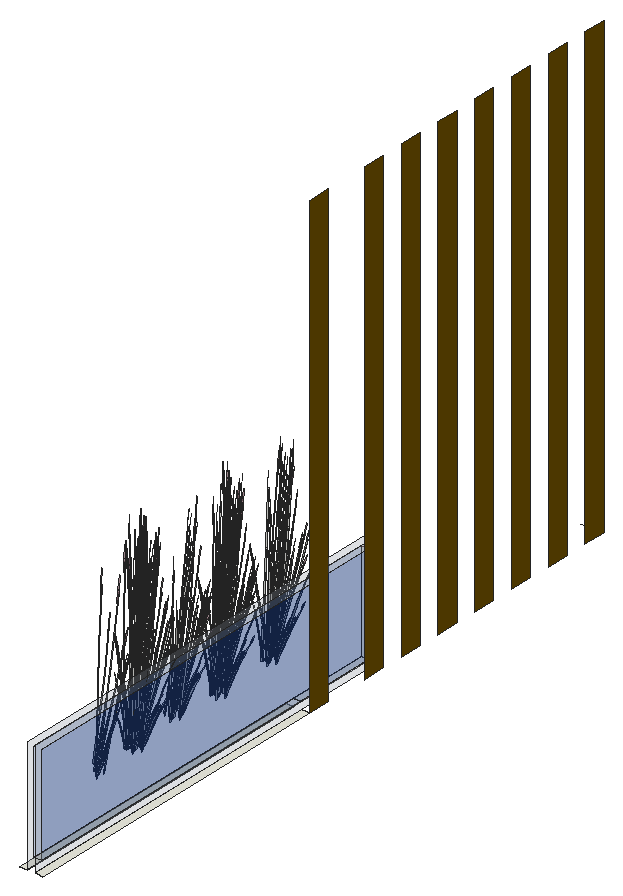
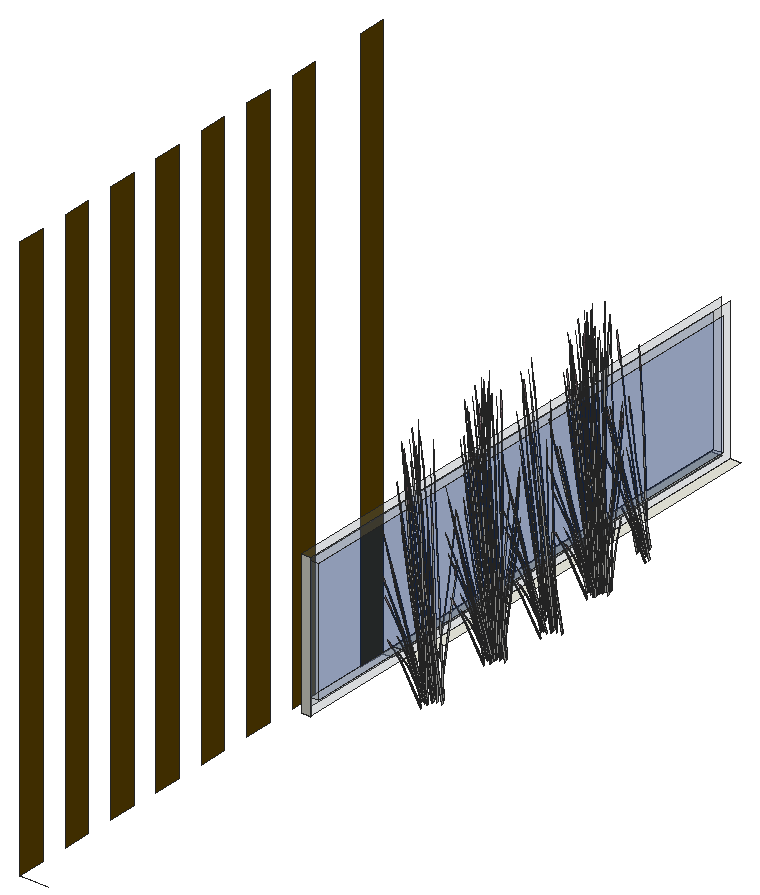
# SketchUp Ruby script. Lengths in inches.
U = 1.inch
M = Sketchup.active_model
def pt(a) = Geom::Point3d.new(a.map { |v| v * U })
def face(e, loops, mat)
  f = e.add_face(loops[0].map { |a| pt(a) })
  loops[1..].each { |l| e.add_face(l.map { |a| pt(a) }).erase! }
  f.material = f.back_material = mat if mat
  f
end
# faces: each face lists its corners as indices into pts; further lists are holes
def faces(e, pts, list, mat = nil) = list.each { |f| face(e, (f[0].is_a?(Array) ? f : [f]).map { |l| l.map { |i| pts[i] } }, mat) }
# xy, xz, yz: faces in a plane at the given z, y or x. An outline is a flat list of corners, or four numbers for a rectangle; further outlines are holes
def ring(l) = l.size == 4 ? [[l[0], l[1]], [l[2], l[1]], [l[2], l[3]], [l[0], l[3]]] : l.each_slice(2).to_a
def flat(e, list, mat, &to3) = list.each { |f| face(e, (f[0].is_a?(Array) ? f : [f]).map { |l| ring(l).map { |u, v| to3.(u, v) } }, mat) }
def xy(e, z, list, mat = nil) = flat(e, list, mat) { |x, y| [x, y, z] }
def xz(e, y, list, mat = nil) = flat(e, list, mat) { |x, z| [x, y, z] }
def yz(e, x, list, mat = nil) = flat(e, list, mat) { |y, z| [x, y, z] }
def lines(e, pts, list) = list.each { |a, b| e.add_line(pt(pts[a]), pt(pts[b])) }
# prism: a flat outline (further loops are holes) pulled along v
def prism(e, loops, v, mat = nil)
  f = face(e, loops, mat); d = Geom::Vector3d.new(v.map { |x| x * U })
  f.pushpull(f.normal.samedirection?(d) ? d.length : -d.length)
end
def box(e, o, s, mat = nil) = prism(e, [[o, [o[0] + s[0], o[1], o[2]], [o[0] + s[0], o[1] + s[1], o[2]], [o[0], o[1] + s[1], o[2]]]], [0, 0, s[2]], mat)
def at(x, y, z, deg = 0) = Geom::Transformation.translation(pt([x, y, z])) * Geom::Transformation.rotation(ORIGIN, Z_AXIS, deg.degrees)
def axes(o, x, y, z) = Geom::Transformation.new([*x, 0, *y, 0, *z, 0, *pt(o).to_a, 1])
def part(name) = M.definitions.add(name)
# library, detail: a bought-in or finely detailed component or shape, given as its bounding box
def library(name, o, s) = part(name).tap { |d| box(d.entities, o, s) }
def detail(e, o, s) = box(e.add_group.entities, o, s)
def put(e, d, t, mat = nil) = e.add_instance(d, t).tap { |i| i.material = mat if mat }
def group(e, t, mat = nil) = e.add_group.tap { |g| g.transformation = t; g.material = mat if mat }.entities
root = M.entities
M.materials.add("D01_Frost_White").color = [238, 238, 227]
M.materials.add("D08_Bronzed_Mustard").color = [102, 74, 0]
M.materials.add("Glass_Basic_01").color = [161, 173, 186]
M.materials["Glass_Basic_01"].alpha = 0.25
M.materials.add("Glass_Sky Reflection_01").color = [0, 46, 142]
M.materials["Glass_Sky Reflection_01"].alpha = 0.25
M.materials.add("LightPink_Translucent").color = [144, 107, 117]
M.materials["LightPink_Translucent"].alpha = 0.75
c1 = part("blade")
p = [[2.15,0.21,22],[0,0.17,0],[0.09,0.45,0],[2.18,0.31,22],[2.29,0.31,22],[0.38,0.45,0],
  [2.48,0.24,33],[2.49,0.24,33],[2.48,0.22,33]]
faces(c1.entities,p,[[0,1,2,3],[4,5,2,3],[6,3,4,7],[8,0,3,6]])
c2 = part("seeds")
p = [[0.3,-0.1,1.38],[-0.01,-0.03,1.59],[-0.01,-0.03,0.03],[0.14,-0.07,-0.07],[0.29,-0.03,3],[0.15,0.01,3.11]]
faces(c2.entities,p,[[0,1,2,3],[1,0,4,5]],"LightPink_Translucent")
c3 = part("blade with seeds")
put(c3.entities,c1,at(0,0,0))
put(c3.entities,c2,axes([2.4,0.25,30.99],[1.5799,-0.05474,1.17369],[-0.12525,1.92788,0.29478],[-0.07173,-0.02425,1.56792]))
xy(root,147,[[310,178,312,265],[314,178,316,265]],"D01_Frost_White")
xy(root,149,[[312,180,314,265],[312,265,314,287]],"Glass_Basic_01")
xz(root,287,[[312,149,314,175]],"Glass_Basic_01")
xz(root,289,[[312,147,314,177]],"D01_Frost_White")
yz(root,312,[[[178,147,289,177],[180,149,287,175]]],"Glass_Basic_01")
yz(root,312,[[180,149,287,175]],"Glass_Sky Reflection_01")
yz(root,314,[[[178,147,289,177],[180,149,287,175]]],"Glass_Basic_01")
yz(root,314,[[180,149,287,175]],"Glass_Sky Reflection_01")
yz(root,316,[[265,147,271,267],[283,147,289,267],[295,147,301,267],[307,147,313,267],[319,147,325,267],
  [331,147,337,267],[343,147,349,267],[355,147,361,267]],"D08_Bronzed_Mustard")
p = [[316,361,147],[310,361,147]]
lines(root,p,[[0,1]])
put(root,c3,axes([300.86,213.89,149.4],[-0.01119,-0.44408,1.19347],[0.50665,0.11511,0.50532],[-0.11983,0.243,1.12654]))
put(root,c3,axes([300.99,214.37,148.77],[0.15027,0.43184,-0.5847],[-0.43285,0.15553,-0.15346],[0.01661,0.14623,1.29063]))
put(root,c3,axes([300.9,215.6,150.95],[0.40438,-0.11212,-0.43168],[0.07074,0.4246,-0.33437],[0.10862,0.12168,0.82598]))
put(root,c3,axes([301.46,216.03,149.25],[-0.26279,-0.01479,0.88755],[0.17355,-0.31417,0.49003],[0.10382,0.11162,0.6962]))
put(root,c3,axes([300.6,215.27,149.1875],[0.00723,-0.15635,1.20808],[0.34559,-0.17464,-0.25981],[0.10668,0.18713,0.51652]))
put(root,c3,axes([299.73,215.9,148.26],[0.06632,-0.02567,1.48974],[0.39894,0.14126,-0.22758],[0.01167,0.15921,0.25375]))
put(root,c3,axes([299.13,215.49,151.23],[0.29336,0.31691,-0.47917],[-0.3099,0.27755,-0.37115],[-0.04464,0.16102,0.91684]))
put(root,c3,axes([298.8125,215.97,149.38],[0.37228,-0.08352,0.05498],[0.08559,0.3365,-0.7291],[-0.0236,0.17034,0.65354]))
put(root,c3,axes([300,215.8,150.95],[0.40284,0.11824,-0.43168],[-0.13808,0.40538,-0.33437],[0.03694,0.16321,0.82598]))
put(root,c3,axes([299.85,215.72,151.21],[0.19559,0.38351,-0.60019],[-0.40262,0.21373,0.07243],[0.04574,0.1853,0.84903]))
put(root,c3,axes([298.98,227.38,149.1875],[-0.11649,0.09547,1.20808],[-0.34886,-0.1671,-0.25981],[0.06467,-0.20781,0.51652]))
put(root,c3,axes([299.27,228.08,151.21],[0.01066,-0.43628,-0.60019],[0.44902,0.0293,0.07243],[0.04739,-0.18483,0.84903]))
put(root,c3,axes([298.55,226.62,149.34],[0.05257,0.27504,0.97034],[-0.29163,-0.15233,0.71294],[0.03138,-0.14083,0.21373]))
put(root,c3,axes([299.17,227.94,150.95],[-0.29336,-0.31691,-0.43168],[0.3099,-0.27755,-0.33437],[0.04464,-0.16102,0.82598]))
put(root,c3,axes([299.8,227.67,148.26],[-0.06134,-0.03716,1.48974],[-0.15755,-0.41512,-0.22758],[0.10629,-0.11265,0.25375]))
put(root,c3,axes([299.79,228.84,151.21],[0.21406,-0.37215,-0.60019],[0.37511,0.26448,0.07243],[0.12781,-0.13483,0.84903]))
put(root,c3,axes([297.48,227.76,149],[-0.25622,-0.47263,0],[0.42866,-0.26357,-0.43598],[0.09763,-0.06003,1.38303]))
put(root,c3,axes([299.78,228.67,150.95],[-0.10528,-0.43067,-0.43168],[0.39868,-0.07534,-0.33437],[0.11425,-0.11568,0.82598]))
put(root,c3,axes([297.83,227.6875,148.7],[0.38354,-0.23583,-0.41945],[0.22925,0.42288,0],[0.08735,-0.05371,1.33059]))
put(root,c3,axes([300.1,228.5,149.1875],[-0.1464,-0.01397,1.20808],[-0.14998,-0.37477,-0.25981],[0.17985,-0.10602,0.51652]))
put(root,c3,axes([298.28,228.65,148.74],[0.27603,-0.35451,-0.52676],[0.34289,0.32147,-0.13825],[0.11061,-0.08844,1.16273]))
put(root,c3,axes([300.27,227.8125,149.34],[-0.1365,0.2401,0.97034],[-0.11733,-0.32258,0.71294],[0.11274,-0.08083,0.21373]))
put(root,c3,axes([297.98,229.06,149.25],[-0.04775,-0.53819,-0.2458],[0.49736,-0.03254,-0.42242],[0.08758,-0.07169,1.34921]))
put(root,c3,axes([297.92,227.875,148.71],[0.38233,0.1167,-0.2617],[-0.09626,0.41098,0.2617],[0.07708,-0.04739,1.17405]))
put(root,c3,axes([298.05,229.49,149.06],[0.46174,0.2286,0.2033],[-0.22222,0.475,0.42242],[0,-0.1095,1.35626]))
put(root,c3,axes([297.9,229.17,149.3],[-0.44501,0.02912,0.37796],[-0.04024,-0.48332,-0.1819],[0.07967,-0.04899,1.2135]))
put(root,c3,axes([299.97,229.625,150.95],[0.11102,-0.42903,-0.43168],[0.38064,0.14706,-0.33437],[0.15325,-0.03934,0.82598]))
put(root,c3,axes([299.37,227.88,149.01],[0.25622,-0.47263,0],[0.42866,0.26357,-0.43598],[0.09763,0.06003,1.38303]))
put(root,c3,axes([300.375,229.75,148.67],[-0.26394,0.0566,1.1961],[-0.04201,-0.45055,0.06846],[0.18486,-0.06819,0.68062]))
put(root,c3,axes([300.86,229.35,148.91],[-0.25407,-0.3016,-0.05481],[0.27826,-0.27635,-0.2485],[0.07884,-0.01946,0.81966]))
put(root,c3,axes([298.53,229.39,148.86],[0,-0.54574,0],[0.51243,0,0],[0,0,1.51605]))
put(root,c3,axes([299.15,228.125,149.09],[-0.38354,-0.23583,0.41945],[0.22925,-0.42288,0],[0.08735,0.05371,1.33059]))
put(root,c3,axes([299.9,229.78,151.21],[0.3601,-0.20831,-0.60019],[0.20068,0.4288,0.07243],[0.17399,-0.04871,0.84903]))
put(root,c3,axes([298.28,229.04,148.99],[-0.33979,0.42804,0.38653],[-0.40368,-0.37784,0.15168],[0.08192,-0.04272,1.34202]))
put(root,c3,axes([297.69,228.34,149.09],[-0.11838,0.46875,0.14904],[-0.43321,-0.13265,0.29641],[0.07483,-0.00228,1.35512]))
put(root,c3,axes([297.51,228.72,148.35],[-0.40337,0.18883,1.08919],[-0.12839,-0.54182,0.42321],[0.24769,0.00901,1.23883]))
put(root,c3,axes([298.6,228.86,149.21],[0.07906,-0.42093,0.12232],[0.38625,0.07307,-0.3493],[0.07029,0.04322,1.07074]))
put(root,c3,axes([300.66,229.45,148.26],[-0.02142,-0.07161,1.48974],[0.14855,-0.41887,-0.22758],[0.14984,-0.00603,0.25375]))
put(root,c3,axes([298.43,228.97,149.3],[-0.24618,-0.39589,0.37796],[0.37289,-0.27878,-0.1819],[0.07967,0.04899,1.2135]))
put(root,c3,axes([298.56,229,149.25],[0.41376,-0.31314,-0.2458],[0.27514,0.44246,-0.42242],[0.10209,0.04493,1.34921]))
put(root,c3,axes([299.6,228.16,148.7],[0.38354,0.23583,-0.41945],[-0.22925,0.42288,0],[0.08735,0.05371,1.33059]))
put(root,c3,axes([298.875,229.51,148.86],[0.45849,0,0],[0,0.4883,0],[0,0,1.50718]))
put(root,c3,axes([299,228.36,149.09],[-0.44036,0.12519,0.14904],[-0.10874,-0.46588,0.29641],[0.03927,0.06788,1.35512]))
put(root,c3,axes([299.49,228.34,148.71],[0.09626,0.41098,-0.2617],[-0.38233,0.1167,0.2617],[0.07708,0.04739,1.17405]))
put(root,c3,axes([298.73,229.26,149.01],[-0.51796,-0.09937,0.41563],[0.10541,-0.56124,0.1631],[0.07569,0.05419,1.44303]))
put(root,c3,axes([298.8125,230.59,148.85],[0.43024,-0.16003,-0.16218],[0.15118,0.46099,0.00007],[0.04749,-0.01769,1.46908]))
put(root,c3,axes([298.86,229.72,148.87],[0.28606,0.30466,0],[-0.28606,0.30466,0],[0,0,1.42996]))
put(root,c3,axes([299.64,229.59,149.09],[-0.32198,-0.34356,0.14904],[0.32447,-0.33323,0.29641],[-0.03556,0.07016,1.35512]))
put(root,c3,axes([299.04,229.07,148.74],[0.42629,0.07733,-0.52676],[-0.08996,0.47699,-0.13825],[0.12722,0.0578,1.16273]))
put(root,c3,axes([300.93,229.9,149.34],[-0.2532,0.07787,0.97034],[0.11918,-0.32181,0.71294],[0.13432,0.02202,0.21373]))
put(root,c3,axes([298.86,229.36,149.3],[0.19883,-0.425,0.37796],[0.41314,0.20454,-0.1819],[0,0.09797,1.2135]))
put(root,c3,axes([298.78,229.6,148.9375],[0,0.54548,-0.04762],[-0.51243,0,0],[0,0.01714,1.5153]))
put(root,c3,axes([298.82,229.22,148.87],[0.24618,0.39589,-0.37796],[-0.37289,0.27878,0.1819],[0.07967,0.04899,1.2135]))
put(root,c3,axes([299.9,229.6,149.09],[0,-0.47166,0.41945],[0.45849,0,0],[0,0.10742,1.33059]))
put(root,c3,axes([299.03,229.46,149.21],[0.38182,-0.13755,0.12232],[0.13371,0.39278,-0.3493],[0,0.08644,1.07074]))
put(root,c3,axes([300.45,230.42,149.1875],[-0.0987,-0.116,1.20808],[0.12841,-0.38374,-0.25981],[0.19968,0.05198,0.51652]))
put(root,c3,axes([298.6875,230.84,148.86],[0.41314,0.21175,0],[-0.19883,0.43999,0],[0,0,1.47801]))
put(root,c3,axes([299.54,230.65,151.21],[0.40965,0.01136,-0.60019],[-0.02751,0.47821,0.07243],[0.17355,0.05047,0.84903]))
put(root,c3,axes([298.54,230.66,148.9375],[0.17817,0.54185,-0.05079],[-0.50909,0.18987,0],[0.00622,0.01892,1.45452]))
put(root,c3,axes([300.21,229.68,149.01],[0.51243,0,0],[0,0.52715,-0.43598],[0,0.12006,1.38303]))
put(root,c3,axes([300.01,229.95,148.86],[-0.51218,-0.00377,-0.04204],[0,-0.52715,0.42192],[-0.0161,0.12,1.33776]))
put(root,c3,axes([298.9,229.49,149.25],[0.46151,0.22505,-0.2458],[-0.22222,0.475,-0.42242],[0.0145,0.11662,1.34921]))
put(root,c3,axes([299.9,230.03,148.71],[-0.28606,0.29428,-0.2617],[-0.28606,-0.29428,0.2617],[0,0.09479,1.17405]))
put(root,c3,axes([298.85,229.84,148.87],[-0.19883,0.425,-0.37796],[-0.41314,-0.20454,0.1819],[0,0.09797,1.2135]))
put(root,c3,axes([300.1,230.04,148.7],[0,0.47166,-0.41945],[-0.45849,0,0],[0,0.10742,1.33059]))
put(root,c3,axes([299.52,231.01,149.34],[-0.23074,-0.13562,0.97034],[0.29794,-0.1378,0.71294],[0.08036,0.11673,0.21373]))
put(root,c3,axes([299.58,231.52,148.26],[0.02986,-0.06809,1.48974],[0.37589,-0.20055,-0.22758],[0.11396,0.1038,0.25375]))
put(root,c3,axes([299.09,229.97,148.77],[0.15027,0.43184,-0.5847],[-0.43285,0.15553,-0.15346],[0.01661,0.14623,1.29063]))
put(root,c3,axes([299,231.2,150.95],[0.40438,-0.11212,-0.43168],[0.07074,0.4246,-0.33437],[0.10862,0.12168,0.82598]))
put(root,c3,axes([299.55,231.63,149.25],[-0.26279,-0.01479,0.88755],[0.17355,-0.31417,0.49003],[0.10382,0.11162,0.6962]))
put(root,c3,axes([298.7,230.87,149.1875],[0.00723,-0.15635,1.20808],[0.34559,-0.17464,-0.25981],[0.10668,0.18713,0.51652]))
put(root,c3,axes([298.1,231.4,150.95],[0.40284,0.11824,-0.43168],[-0.13808,0.40538,-0.33437],[0.03694,0.16321,0.82598]))
put(root,c3,axes([297.95,231.32,151.21],[0.19559,0.38351,-0.60019],[-0.40262,0.21373,0.07243],[0.04574,0.1853,0.84903]))
put(root,c3,axes([297.57,242.83,148.26],[-0.06134,-0.03716,1.48974],[-0.15755,-0.41512,-0.22758],[0.10629,-0.11265,0.25375]))
put(root,c3,axes([297.5625,244,151.21],[0.21406,-0.37215,-0.60019],[0.37511,0.26448,0.07243],[0.12781,-0.13483,0.84903]))
put(root,c3,axes([297.55,243.83,150.95],[-0.10528,-0.43067,-0.43168],[0.39868,-0.07534,-0.33437],[0.11425,-0.11568,0.82598]))
put(root,c3,axes([297.875,243.66,149.1875],[-0.1464,-0.01397,1.20808],[-0.14998,-0.37477,-0.25981],[0.17985,-0.10602,0.51652]))
put(root,c3,axes([296.05,243.82,148.74],[0.27603,-0.35451,-0.52676],[0.34289,0.32147,-0.13825],[0.11061,-0.08844,1.16273]))
put(root,c3,axes([298.04,242.97,149.34],[-0.1365,0.2401,0.97034],[-0.11733,-0.32258,0.71294],[0.11274,-0.08083,0.21373]))
put(root,c3,axes([297.74,244.79,150.95],[0.11102,-0.42903,-0.43168],[0.38064,0.14706,-0.33437],[0.15325,-0.03934,0.82598]))
put(root,c3,axes([297.14,243.04,149.01],[0.25622,-0.47263,0],[0.42866,0.26357,-0.43598],[0.09763,0.06003,1.38303]))
put(root,c3,axes([298.14,244.91,148.67],[-0.26394,0.0566,1.1961],[-0.04201,-0.45055,0.06846],[0.18486,-0.06819,0.68062]))
put(root,c3,axes([298.625,244.51,148.91],[-0.25407,-0.3016,-0.05481],[0.27826,-0.27635,-0.2485],[0.07884,-0.01946,0.81966]))
put(root,c3,axes([297.67,244.94,151.21],[0.3601,-0.20831,-0.60019],[0.20068,0.4288,0.07243],[0.17399,-0.04871,0.84903]))
put(root,c3,axes([295.28,243.88,148.35],[-0.40337,0.18883,1.08919],[-0.12839,-0.54182,0.42321],[0.24769,0.00901,1.23883]))
put(root,c3,axes([298.43,244.61,148.26],[-0.02142,-0.07161,1.48974],[0.14855,-0.41887,-0.22758],[0.14984,-0.00603,0.25375]))
put(root,c3,axes([296.33,244.16,149.25],[0.41376,-0.31314,-0.2458],[0.27514,0.44246,-0.42242],[0.10209,0.04493,1.34921]))
put(root,c3,axes([297.37,243.33,148.7],[0.38354,0.23583,-0.41945],[-0.22925,0.42288,0],[0.08735,0.05371,1.33059]))
put(root,c3,axes([297.26,243.5,148.71],[0.09626,0.41098,-0.2617],[-0.38233,0.1167,0.2617],[0.07708,0.04739,1.17405]))
put(root,c3,axes([296.8125,244.23,148.74],[0.42629,0.07733,-0.52676],[-0.08996,0.47699,-0.13825],[0.12722,0.0578,1.16273]))
put(root,c3,axes([298.69,245.0625,149.34],[-0.2532,0.07787,0.97034],[0.11918,-0.32181,0.71294],[0.13432,0.02202,0.21373]))
put(root,c3,axes([298.22,245.58,149.1875],[-0.0987,-0.116,1.20808],[0.12841,-0.38374,-0.25981],[0.19968,0.05198,0.51652]))
put(root,c3,axes([297.3125,245.8125,151.21],[0.40965,0.01136,-0.60019],[-0.02751,0.47821,0.07243],[0.17355,0.05047,0.84903]))
put(root,c3,axes([297.98,244.84,149.01],[0.51243,0,0],[0,0.52715,-0.43598],[0,0.12006,1.38303]))
put(root,c3,axes([297.56,246.01,150.82],[0.23317,0.29531,-0.29918],[-0.26625,0.27955,0.38624],[0.13527,0.04253,0.73904]))
put(root,c3,axes([297.29,246.18,149.34],[-0.23074,-0.13562,0.97034],[0.29794,-0.1378,0.71294],[0.08036,0.11673,0.21373]))
put(root,c3,axes([297.35,246.68,148.26],[0.02986,-0.06809,1.48974],[0.37589,-0.20055,-0.22758],[0.11396,0.1038,0.25375]))
put(root,c3,axes([296.76,246.36,150.95],[0.40438,-0.11212,-0.43168],[0.07074,0.4246,-0.33437],[0.10862,0.12168,0.82598]))
put(root,c3,axes([297.32,246.79,149.25],[-0.26279,-0.01479,0.88755],[0.17355,-0.31417,0.49003],[0.10382,0.11162,0.6962]))
put(root,c3,axes([296.46,246.03,149.1875],[0.00723,-0.15635,1.20808],[0.34559,-0.17464,-0.25981],[0.10668,0.18713,0.51652]))
put(root,c3,axes([298.22,255.59,149.1875],[-0.11649,0.09547,1.20808],[-0.34886,-0.1671,-0.25981],[0.06467,-0.20781,0.51652]))
put(root,c3,axes([298.51,256.29,151.21],[0.01066,-0.43628,-0.60019],[0.44902,0.0293,0.07243],[0.04739,-0.18483,0.84903]))
put(root,c3,axes([298.42,256.15,150.95],[-0.29336,-0.31691,-0.43168],[0.3099,-0.27755,-0.33437],[0.04464,-0.16102,0.82598]))
put(root,c3,axes([298.69,256.03,150.82],[0.27728,-0.24833,-0.29918],[0.26248,0.28355,0.38624],[0.03994,-0.14407,0.73904]))
put(root,c3,axes([299.04,255.88,148.26],[-0.06134,-0.03716,1.48974],[-0.15755,-0.41512,-0.22758],[0.10629,-0.11265,0.25375]))
put(root,c3,axes([299.04,257.05,151.21],[0.21406,-0.37215,-0.60019],[0.37511,0.26448,0.07243],[0.12781,-0.13483,0.84903]))
put(root,c3,axes([299.03,256.88,150.95],[-0.10528,-0.43067,-0.43168],[0.39868,-0.07534,-0.33437],[0.11425,-0.11568,0.82598]))
put(root,c3,axes([297.07,255.9,148.7],[0.38354,-0.23583,-0.41945],[0.22925,0.42288,0],[0.08735,-0.05371,1.33059]))
put(root,c3,axes([299.35,256.71,149.1875],[-0.1464,-0.01397,1.20808],[-0.14998,-0.37477,-0.25981],[0.17985,-0.10602,0.51652]))
put(root,c3,axes([297.53,256.86,148.74],[0.27603,-0.35451,-0.52676],[0.34289,0.32147,-0.13825],[0.11061,-0.08844,1.16273]))
put(root,c3,axes([299.52,256.02,149.34],[-0.1365,0.2401,0.97034],[-0.11733,-0.32258,0.71294],[0.11274,-0.08083,0.21373]))
put(root,c3,axes([299.32,256.92,150.82],[0.35672,-0.06741,-0.29918],[0.09419,0.38534,0.38624],[0.10222,-0.1035,0.73904]))
put(root,c3,axes([297.23,257.27,149.25],[-0.04775,-0.53819,-0.2458],[0.49736,-0.03254,-0.42242],[0.08758,-0.07169,1.34921]))
put(root,c3,axes([297.16,256.08,148.71],[0.38233,0.1167,-0.2617],[-0.09626,0.41098,0.2617],[0.07708,-0.04739,1.17405]))
put(root,c3,axes([299.21,257.84,150.95],[0.11102,-0.42903,-0.43168],[0.38064,0.14706,-0.33437],[0.15325,-0.03934,0.82598]))
put(root,c3,axes([298.61,256.09,149.01],[0.25622,-0.47263,0],[0.42866,0.26357,-0.43598],[0.09763,0.06003,1.38303]))
put(root,c3,axes([299.62,257.96,148.67],[-0.26394,0.0566,1.1961],[-0.04201,-0.45055,0.06846],[0.18486,-0.06819,0.68062]))
put(root,c3,axes([300.1,257.56,148.91],[-0.25407,-0.3016,-0.05481],[0.27826,-0.27635,-0.2485],[0.07884,-0.01946,0.81966]))
put(root,c3,axes([298.39,256.34,149.09],[-0.38354,-0.23583,0.41945],[0.22925,-0.42288,0],[0.08735,0.05371,1.33059]))
put(root,c3,axes([299.14,257.99,151.21],[0.3601,-0.20831,-0.60019],[0.20068,0.4288,0.07243],[0.17399,-0.04871,0.84903]))
put(root,c3,axes([297.52,257.25,148.99],[-0.33979,0.42804,0.38653],[-0.40368,-0.37784,0.15168],[0.08192,-0.04272,1.34202]))
put(root,c3,axes([296.76,256.93,148.35],[-0.40337,0.18883,1.08919],[-0.12839,-0.54182,0.42321],[0.24769,0.00901,1.23883]))
put(root,c3,axes([297.84,257.07,149.21],[0.07906,-0.42093,0.12232],[0.38625,0.07307,-0.3493],[0.07029,0.04322,1.07074]))
put(root,c3,axes([299.91,257.66,148.26],[-0.02142,-0.07161,1.48974],[0.14855,-0.41887,-0.22758],[0.14984,-0.00603,0.25375]))
put(root,c3,axes([297.67,257.18,149.3],[-0.24618,-0.39589,0.37796],[0.37289,-0.27878,-0.1819],[0.07967,0.04899,1.2135]))
put(root,c3,axes([297.8,257.21,149.25],[0.41376,-0.31314,-0.2458],[0.27514,0.44246,-0.42242],[0.10209,0.04493,1.34921]))
put(root,c3,axes([299.45,258.03,150.82],[0.34057,0.13158,-0.29918],[-0.09933,0.38387,0.38624],[0.13712,-0.0352,0.73904]))
put(root,c3,axes([298.84,256.375,148.7],[0.38354,0.23583,-0.41945],[-0.22925,0.42288,0],[0.08735,0.05371,1.33059]))
put(root,c3,axes([298.12,257.72,148.86],[0.45849,0,0],[0,0.4883,0],[0,0,1.50718]))
put(root,c3,axes([298.74,256.55,148.71],[0.09626,0.41098,-0.2617],[-0.38233,0.1167,0.2617],[0.07708,0.04739,1.17405]))
put(root,c3,axes([297.97,257.47,149.01],[-0.51796,-0.09937,0.41563],[0.10541,-0.56124,0.1631],[0.07569,0.05419,1.44303]))
put(root,c3,axes([298.05,258.8,148.85],[0.43024,-0.16003,-0.16218],[0.15118,0.46099,0.00007],[0.04749,-0.01769,1.46908]))
put(root,c3,axes([298.11,257.93,148.87],[0.28606,0.30466,0],[-0.28606,0.30466,0],[0,0,1.42996]))
put(root,c3,axes([298.28,257.28,148.74],[0.42629,0.07733,-0.52676],[-0.08996,0.47699,-0.13825],[0.12722,0.0578,1.16273]))
put(root,c3,axes([300.17,258.11,149.34],[-0.2532,0.07787,0.97034],[0.11918,-0.32181,0.71294],[0.13432,0.02202,0.21373]))
put(root,c3,axes([298.1,257.57,149.3],[0.19883,-0.425,0.37796],[0.41314,0.20454,-0.1819],[0,0.09797,1.2135]))
put(root,c3,axes([298.0625,257.43,148.87],[0.24618,0.39589,-0.37796],[-0.37289,0.27878,0.1819],[0.07967,0.04899,1.2135]))
put(root,c3,axes([299.15,257.81,149.09],[0,-0.47166,0.41945],[0.45849,0,0],[0,0.10742,1.33059]))
put(root,c3,axes([298.27,257.67,149.21],[0.38182,-0.13755,0.12232],[0.13371,0.39278,-0.3493],[0,0.08644,1.07074]))
put(root,c3,axes([299.69,258.625,149.1875],[-0.0987,-0.116,1.20808],[0.12841,-0.38374,-0.25981],[0.19968,0.05198,0.51652]))
put(root,c3,axes([297.93,259.05,148.86],[0.41314,0.21175,0],[-0.19883,0.43999,0],[0,0,1.47801]))
put(root,c3,axes([298.79,258.86,151.21],[0.40965,0.01136,-0.60019],[-0.02751,0.47821,0.07243],[0.17355,0.05047,0.84903]))
put(root,c3,axes([299.46,257.89,149.01],[0.51243,0,0],[0,0.52715,-0.43598],[0,0.12006,1.38303]))
put(root,c3,axes([298.14,257.7,149.25],[0.46151,0.22505,-0.2458],[-0.22222,0.475,-0.42242],[0.0145,0.11662,1.34921]))
put(root,c3,axes([299.03,259.06,150.82],[0.23317,0.29531,-0.29918],[-0.26625,0.27955,0.38624],[0.13527,0.04253,0.73904]))
put(root,c3,axes([299.15,258.24,148.71],[-0.28606,0.29428,-0.2617],[-0.28606,-0.29428,0.2617],[0,0.09479,1.17405]))
put(root,c3,axes([299.34,258.25,148.7],[0,0.47166,-0.41945],[-0.45849,0,0],[0,0.10742,1.33059]))
put(root,c3,axes([298.76,259.22,149.34],[-0.23074,-0.13562,0.97034],[0.29794,-0.1378,0.71294],[0.08036,0.11673,0.21373]))
put(root,c3,axes([298.82,259.73,148.26],[0.02986,-0.06809,1.48974],[0.37589,-0.20055,-0.22758],[0.11396,0.1038,0.25375]))
put(root,c3,axes([298.33,258.18,148.77],[0.15027,0.43184,-0.5847],[-0.43285,0.15553,-0.15346],[0.01661,0.14623,1.29063]))
put(root,c3,axes([298.24,259.41,150.95],[0.40438,-0.11212,-0.43168],[0.07074,0.4246,-0.33437],[0.10862,0.12168,0.82598]))
put(root,c3,axes([298.8,259.84,149.25],[-0.26279,-0.01479,0.88755],[0.17355,-0.31417,0.49003],[0.10382,0.11162,0.6962]))
put(root,c3,axes([297.9375,259.08,149.1875],[0.00723,-0.15635,1.20808],[0.34559,-0.17464,-0.25981],[0.10668,0.18713,0.51652]))
put(root,c3,axes([297.34,259.61,150.95],[0.40284,0.11824,-0.43168],[-0.13808,0.40538,-0.33437],[0.03694,0.16321,0.82598]))
put(root,c3,axes([297.51,273.19,149.1875],[-0.11649,0.09547,1.20808],[-0.34886,-0.1671,-0.25981],[0.06467,-0.20781,0.51652]))
put(root,c3,axes([297.79,273.9,151.21],[0.01066,-0.43628,-0.60019],[0.44902,0.0293,0.07243],[0.04739,-0.18483,0.84903]))
put(root,c3,axes([298.32,273.49,148.26],[-0.06134,-0.03716,1.48974],[-0.15755,-0.41512,-0.22758],[0.10629,-0.11265,0.25375]))
put(root,c3,axes([298.32,274.66,151.21],[0.21406,-0.37215,-0.60019],[0.37511,0.26448,0.07243],[0.12781,-0.13483,0.84903]))
put(root,c3,axes([298.3125,274.49,150.95],[-0.10528,-0.43067,-0.43168],[0.39868,-0.07534,-0.33437],[0.11425,-0.11568,0.82598]))
put(root,c3,axes([296.36,273.5,148.7],[0.38354,-0.23583,-0.41945],[0.22925,0.42288,0],[0.08735,-0.05371,1.33059]))
put(root,c3,axes([298.63,274.32,149.1875],[-0.1464,-0.01397,1.20808],[-0.14998,-0.37477,-0.25981],[0.17985,-0.10602,0.51652]))
put(root,c3,axes([296.8125,274.47,148.74],[0.27603,-0.35451,-0.52676],[0.34289,0.32147,-0.13825],[0.11061,-0.08844,1.16273]))
put(root,c3,axes([298.8,273.63,149.34],[-0.1365,0.2401,0.97034],[-0.11733,-0.32258,0.71294],[0.11274,-0.08083,0.21373]))
put(root,c3,axes([298.5,275.44,150.95],[0.11102,-0.42903,-0.43168],[0.38064,0.14706,-0.33437],[0.15325,-0.03934,0.82598]))
put(root,c3,axes([297.89,273.69,149.01],[0.25622,-0.47263,0],[0.42866,0.26357,-0.43598],[0.09763,0.06003,1.38303]))
put(root,c3,axes([298.9,275.5625,148.67],[-0.26394,0.0566,1.1961],[-0.04201,-0.45055,0.06846],[0.18486,-0.06819,0.68062]))
put(root,c3,axes([299.38,275.16,148.91],[-0.25407,-0.3016,-0.05481],[0.27826,-0.27635,-0.2485],[0.07884,-0.01946,0.81966]))
put(root,c3,axes([297.67,273.94,149.09],[-0.38354,-0.23583,0.41945],[0.22925,-0.42288,0],[0.08735,0.05371,1.33059]))
put(root,c3,axes([298.42,275.6,151.21],[0.3601,-0.20831,-0.60019],[0.20068,0.4288,0.07243],[0.17399,-0.04871,0.84903]))
put(root,c3,axes([296.04,274.53,148.35],[-0.40337,0.18883,1.08919],[-0.12839,-0.54182,0.42321],[0.24769,0.00901,1.23883]))
put(root,c3,axes([297.125,274.68,149.21],[0.07906,-0.42093,0.12232],[0.38625,0.07307,-0.3493],[0.07029,0.04322,1.07074]))
put(root,c3,axes([299.19,275.27,148.26],[-0.02142,-0.07161,1.48974],[0.14855,-0.41887,-0.22758],[0.14984,-0.00603,0.25375]))
put(root,c3,axes([297.09,274.8125,149.25],[0.41376,-0.31314,-0.2458],[0.27514,0.44246,-0.42242],[0.10209,0.04493,1.34921]))
put(root,c3,axes([298.13,273.98,148.7],[0.38354,0.23583,-0.41945],[-0.22925,0.42288,0],[0.08735,0.05371,1.33059]))
put(root,c3,axes([298.02,274.16,148.71],[0.09626,0.41098,-0.2617],[-0.38233,0.1167,0.2617],[0.07708,0.04739,1.17405]))
put(root,c3,axes([297.34,276.4,148.85],[0.43024,-0.16003,-0.16218],[0.15118,0.46099,0.00007],[0.04749,-0.01769,1.46908]))
put(root,c3,axes([297.57,274.88,148.74],[0.42629,0.07733,-0.52676],[-0.08996,0.47699,-0.13825],[0.12722,0.0578,1.16273]))
put(root,c3,axes([299.45,275.72,149.34],[-0.2532,0.07787,0.97034],[0.11918,-0.32181,0.71294],[0.13432,0.02202,0.21373]))
put(root,c3,axes([297.35,275.03,148.87],[0.24618,0.39589,-0.37796],[-0.37289,0.27878,0.1819],[0.07967,0.04899,1.2135]))
put(root,c3,axes([298.43,275.41,149.09],[0,-0.47166,0.41945],[0.45849,0,0],[0,0.10742,1.33059]))
put(root,c3,axes([298.98,276.23,149.1875],[-0.0987,-0.116,1.20808],[0.12841,-0.38374,-0.25981],[0.19968,0.05198,0.51652]))
put(root,c3,axes([298.07,276.47,151.21],[0.40965,0.01136,-0.60019],[-0.02751,0.47821,0.07243],[0.17355,0.05047,0.84903]))
put(root,c3,axes([298.74,275.49,149.01],[0.51243,0,0],[0,0.52715,-0.43598],[0,0.12006,1.38303]))
put(root,c3,axes([298.625,275.85,148.7],[0,0.47166,-0.41945],[-0.45849,0,0],[0,0.10742,1.33059]))
put(root,c3,axes([298.04,276.83,149.34],[-0.23074,-0.13562,0.97034],[0.29794,-0.1378,0.71294],[0.08036,0.11673,0.21373]))
put(root,c3,axes([298.11,277.33,148.26],[0.02986,-0.06809,1.48974],[0.37589,-0.20055,-0.22758],[0.11396,0.1038,0.25375]))
put(root,c3,axes([297.52,277.02,150.95],[0.40438,-0.11212,-0.43168],[0.07074,0.4246,-0.33437],[0.10862,0.12168,0.82598]))
put(root,c3,axes([298.08,277.45,149.25],[-0.26279,-0.01479,0.88755],[0.17355,-0.31417,0.49003],[0.10382,0.11162,0.6962]))
put(root,c3,axes([297.22,276.6875,149.1875],[0.00723,-0.15635,1.20808],[0.34559,-0.17464,-0.25981],[0.10668,0.18713,0.51652]))
